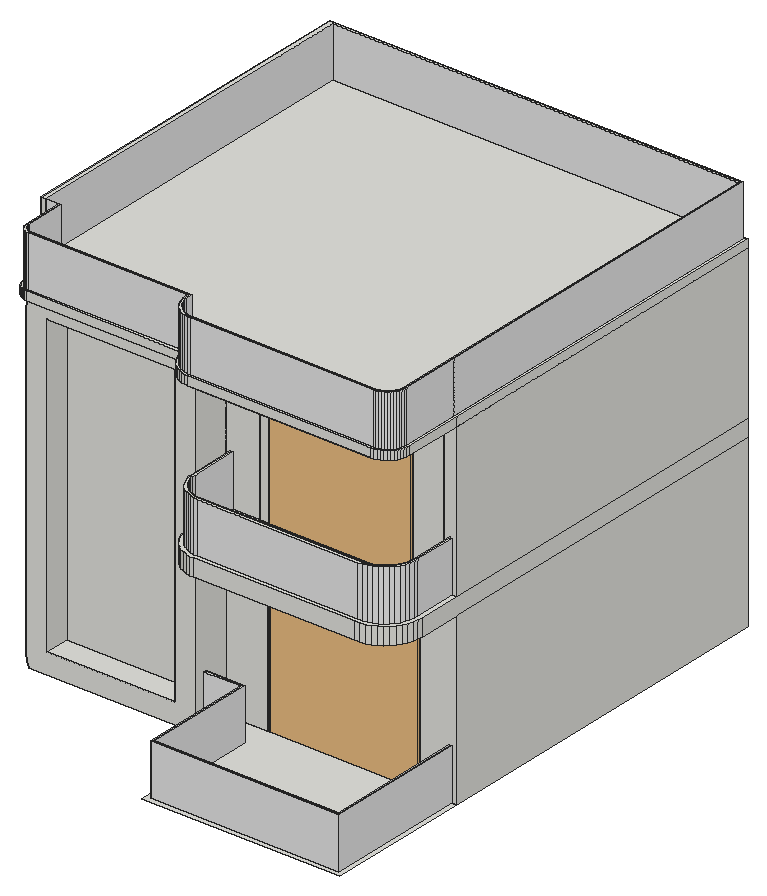
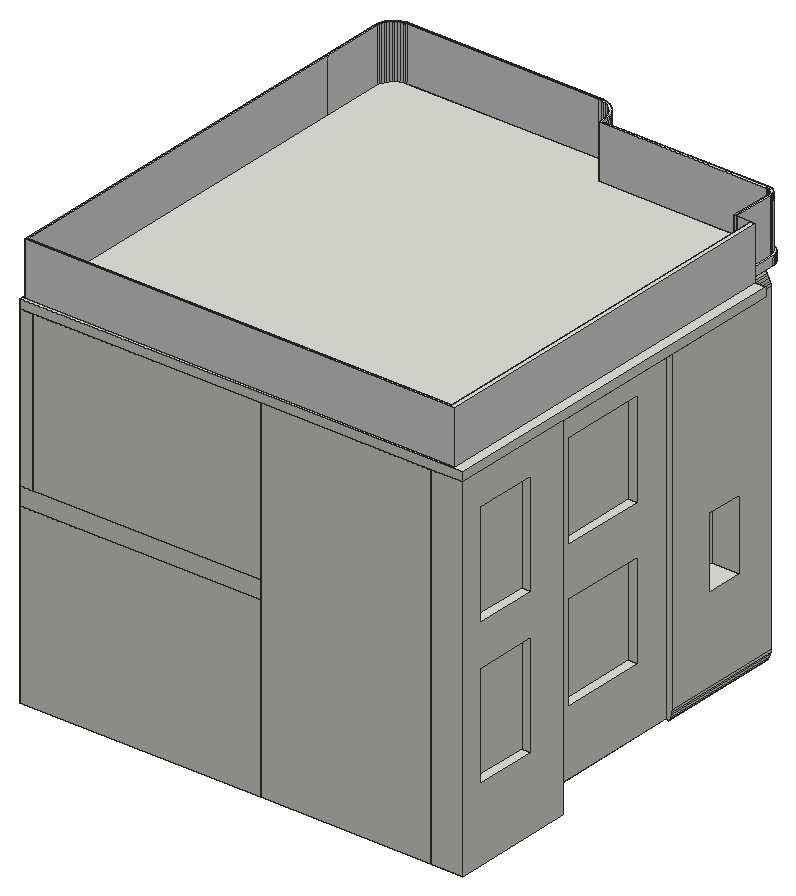
# SketchUp Ruby script. Lengths in inches.
U = 1.inch
M = Sketchup.active_model
def pt(a) = Geom::Point3d.new(a.map { |v| v * U })
def face(e, loops, mat)
  f = e.add_face(loops[0].map { |a| pt(a) })
  loops[1..].each { |l| e.add_face(l.map { |a| pt(a) }).erase! }
  f.material = f.back_material = mat if mat
  f
end
# faces: each face lists its corners as indices into pts; further lists are holes
def faces(e, pts, list, mat = nil) = list.each { |f| face(e, (f[0].is_a?(Array) ? f : [f]).map { |l| l.map { |i| pts[i] } }, mat) }
# xy, xz, yz: faces in a plane at the given z, y or x. An outline is a flat list of corners, or four numbers for a rectangle; further outlines are holes
def ring(l) = l.size == 4 ? [[l[0], l[1]], [l[2], l[1]], [l[2], l[3]], [l[0], l[3]]] : l.each_slice(2).to_a
def flat(e, list, mat, &to3) = list.each { |f| face(e, (f[0].is_a?(Array) ? f : [f]).map { |l| ring(l).map { |u, v| to3.(u, v) } }, mat) }
def xy(e, z, list, mat = nil) = flat(e, list, mat) { |x, y| [x, y, z] }
def xz(e, y, list, mat = nil) = flat(e, list, mat) { |x, z| [x, y, z] }
def yz(e, x, list, mat = nil) = flat(e, list, mat) { |y, z| [x, y, z] }
def lines(e, pts, list) = list.each { |a, b| e.add_line(pt(pts[a]), pt(pts[b])) }
# prism: a flat outline (further loops are holes) pulled along v
def prism(e, loops, v, mat = nil)
  f = face(e, loops, mat); d = Geom::Vector3d.new(v.map { |x| x * U })
  f.pushpull(f.normal.samedirection?(d) ? d.length : -d.length)
end
def box(e, o, s, mat = nil) = prism(e, [[o, [o[0] + s[0], o[1], o[2]], [o[0] + s[0], o[1] + s[1], o[2]], [o[0], o[1] + s[1], o[2]]]], [0, 0, s[2]], mat)
def at(x, y, z, deg = 0) = Geom::Transformation.translation(pt([x, y, z])) * Geom::Transformation.rotation(ORIGIN, Z_AXIS, deg.degrees)
def axes(o, x, y, z) = Geom::Transformation.new([*x, 0, *y, 0, *z, 0, *pt(o).to_a, 1])
def part(name) = M.definitions.add(name)
# library, detail: a bought-in or finely detailed component or shape, given as its bounding box
def library(name, o, s) = part(name).tap { |d| box(d.entities, o, s) }
def detail(e, o, s) = box(e.add_group.entities, o, s)
def put(e, d, t, mat = nil) = e.add_instance(d, t).tap { |i| i.material = mat if mat }
def group(e, t, mat = nil) = e.add_group.tap { |g| g.transformation = t; g.material = mat if mat }.entities
root = M.entities
M.materials.add("[Mirror 02]").color = [229, 229, 229]
c1 = library("Curtains 004",[-15.59,-2.26,0],[31.18,4.52,116.91])
c2 = library("Door 46-41",[-69.27,-3.71,0.02],[138.54,7.43,97.71])
xy(root,252,[[219.5625,0,360,0,360,102.93,356.5,102.93,356.5,3.5,223.0625,3.5,223.0625,83,196.57,83,196.57,79.5,219.5625,79.5],[223.0625,3.5,223.0625,83,196.57,83,196.57,84.76,224.82,84.76,224.82,5.26,354.74,5.26,354.74,102.93,356.5,102.93,356.5,3.5],[224.82,5.26,354.74,5.26,354.74,102.93,334.22,102.93,334.22,111.93,227.87,111.93,227.87,102.93,196.57,102.93,196.57,84.76,224.82,84.76],[196.57,102.93,196.57,360,360,360,360,102.93,334.22,102.93,334.22,111.93,351,111.93,351,351,205.57,351,205.57,111.93,227.87,111.93,227.87,102.93],[205.57,111.93,351,351],
  [81,159.75,196.57,275],[59.04,275,81,360],[81,275,196.57,360]])
xy(root,266.67,[[91.49,76.3125,181.9,93.625]])
xy(root,288,[[223.0625,3.5,356.5,3.5,356.5,102.93,354.74,102.93,354.74,5.26,224.82,5.26,224.82,84.76,196.57,84.76,196.57,83,223.0625,83]])
xy(root,296.33,[[81,184.12,87.625,242.93]])
xy(root,301.73,[[59.04,301.97,65.66,345.47]])
xy(root,316.9,[[76.8125,102.66,95.5625,128.53]])
xy(root,361.83,[[81,184.12,87.625,242.93]])
xy(root,365.21,[[76.8125,102.66,95.5625,128.53]])
xy(root,372,[[219.65,46.1875,216.64,46.38,213.67,46.97,210.82,47.94,208.11,49.28,205.6,50.96,203.33,52.95,201.34,55.22,199.66,57.73,198.33,60.43,197.36,63.29,196.77,66.25,196.57,69.27,196.57,102.93,227.87,102.93,227.87,111.93,205.57,111.93,205.57,351,351,351,351,111.93,334.22,111.93,334.22,102.93,360,102.93,360,72.79,359.77,69.32,359.09,65.9,357.98,62.61,356.4375,59.49,354.5,56.6,352.21,53.98,349.59,51.68,346.7,49.75,343.58,48.21,340.28,47.09,336.87,46.42,333.4,46.1875],[196.57,102.93,196.57,360,360,360,360,102.93,334.22,102.93,334.22,111.93,351,111.93,351,351,205.57,351,205.57,111.93,227.87,111.93,227.87,102.93]])
xy(root,372.12,[[59.04,301.97,65.66,345.47]])
xy(root,384,[[219.65,46.1875,333.4,46.1875,336.87,46.42,340.28,47.09,343.58,48.21,346.7,49.75,349.59,51.68,352.21,53.98,354.5,56.6,356.4375,59.49,357.98,62.61,359.09,65.9,359.77,69.32,360,72.79,360,102.8125,356.95,102.8125,356.95,72.79,356.74,69.72,356.14,66.69,355.15,63.78,353.79,61.02,352.08,58.45,350.05,56.14,347.73,54.11,345.17,52.4,342.41,51.03,339.49,50.04,336.47,49.44,333.4,49.24,219.65,49.24,217.03,49.41,214.47,49.92,211.98,50.77,209.64,51.92,207.46,53.38,205.49,55.11,203.76,57.08,202.31,59.25,201.15,61.6,200.31,64.08,199.79,66.65,199.625,69.27,199.625,102.8125,196.57,102.8125,196.57,69.27,196.77,66.25,197.36,63.29,198.33,60.43,199.66,57.73,201.34,55.22,203.33,52.95,205.6,50.96,208.11,49.28,210.82,47.94,213.67,46.97,216.64,46.38],[219.65,49.24,217.03,49.41,214.47,49.92,211.98,50.77,209.64,51.92,207.46,53.38,205.49,55.11,203.76,57.08,202.31,59.25,201.15,61.6,200.31,64.08,199.79,66.65,199.625,69.27,199.625,102.8125,201.5,102.8125,201.5,69.27,201.66,66.9,202.12,64.57,202.89,62.32,203.94,60.19,205.25,58.22,206.82,56.4375,208.6,54.87,210.58,53.55,212.7,52.5,214.95,51.74,217.28,51.28,219.65,51.12,333.4,51.12,336.23,51.31,339.01,51.86,341.69,52.77,344.23,54.02,346.59,55.6,348.72,57.47,350.59,59.6,352.16,61.96,353.42,64.5,354.33,67.18,354.88,69.96,355.07,72.79,355.07,102.8125,356.95,102.8125,356.95,72.79,356.74,69.72,356.14,66.69,355.15,63.78,353.79,61.02,352.08,58.45,350.05,56.14,347.73,54.11,345.17,52.4,342.41,51.03,339.49,50.04,336.47,49.44,333.4,49.24],[219.65,51.12,333.4,51.12,336.23,51.31,339.01,51.86,341.69,52.77,344.23,54.02,346.59,55.6,348.72,57.47,350.59,59.6,352.16,61.96,353.42,64.5,354.33,67.18,354.88,69.96,355.07,72.79,355.07,102.8125,329.25,102.8125,329.25,111.8125,227.25,111.8125,227.25,102.8125,201.5,102.8125,201.5,69.27,201.66,66.9,202.12,64.57,202.89,62.32,203.94,60.19,205.25,58.22,206.82,56.4375,208.6,54.87,210.58,53.55,212.7,52.5,214.95,51.74,217.28,51.28],[196.57,102.8125,227.25,111.8125],[329.25,102.8125,351,111.8125],
  [351,102.8125,360,360],[196.57,111.8125,351,351],[196.57,351,351,360]])
xy(root,394.46,[[81,184.12,87.625,242.93]])
xy(root,399.98,[[59.04,301.97,65.66,345.47]])
xy(root,420,[[219.65,49.24,333.4,49.24,336.47,49.44,339.49,50.04,342.41,51.03,345.17,52.4,347.73,54.11,350.05,56.14,352.08,58.45,353.79,61.02,355.15,63.78,356.14,66.69,356.74,69.72,356.95,72.79,356.95,102.8125,355.07,102.8125,355.07,72.79,354.88,69.96,354.33,67.18,353.42,64.5,352.16,61.96,350.59,59.6,348.72,57.47,346.59,55.6,344.23,54.02,341.69,52.77,339.01,51.86,336.23,51.31,333.4,51.12,219.65,51.12,217.28,51.28,214.95,51.74,212.7,52.5,210.58,53.55,208.6,54.87,206.82,56.4375,205.25,58.22,203.94,60.19,202.89,62.32,202.12,64.57,201.66,66.9,201.5,69.27,201.5,102.8125,199.625,102.8125,199.625,69.27,199.79,66.65,200.31,64.08,201.15,61.6,202.31,59.25,203.76,57.08,205.49,55.11,207.46,53.38,209.64,51.92,211.98,50.77,214.47,49.92,217.03,49.41]])
xy(root,459.96,[[81,184.12,87.625,242.93]])
xy(root,470.37,[[59.04,301.97,65.66,345.47]])
xy(root,474.75,[[227.25,102.8125,329.25,111.8125]])
xy(root,477.33,[[91.49,76.3125,181.9,93.625]])
xy(root,492,[[215.57,46.1875,213.09,46.35,210.65,46.83,208.3,47.63,206.07,48.73,204,50.11,202.13,51.75,200.5,53.62,199.12,55.6875,198.02,57.91,197.22,60.27,196.73,62.71,196.57,65.18,85.88,65.18,84.7,65.26,83.54,65.49,82.41,65.875,81.35,66.4,80.36,67.06,79.47,67.84,78.6875,68.73,78.03,69.72,77.5,70.78,77.12,71.91,76.89,73.07,76.8125,74.26,76.8125,102.8125,88.75,102.8125,88.75,76.3125,184.95,76.3125,184.95,102.8125,351,102.8125,351,47.44,350.77,47.33,348.91,46.7,347,46.32,345.04,46.1875],[351,47.44,351,102.8125,360,102.8125,360,61.14,359.87,59.19,359.49,57.27,358.86,55.42,358,53.67,356.91,52.04,355.62,50.57,354.15,49.28,352.52,48.19],[88.75,76.3125,184.95,102.8125],[88.75,76.3125,184.95,102.8125],[59.04,102.8125,88.75,111.8125],
  [88.75,102.8125,184.95,111.8125],[184.95,102.8125,196.57,111.8125],[196.57,102.8125,351,111.8125],[351,102.8125,360,360],[59.04,111.8125,88.75,159.75],
  [88.75,111.8125,184.95,159.75],[184.95,111.8125,184.95,159.75,196.57,159.75,196.57,351,351,351,351,111.8125],[59.04,159.75,81,275],[81,159.75,196.57,275],[59.04,275,81,351],
  [81,275,196.57,351],[59.04,351,81,360],[81,351,196.57,360],[196.57,351,351,360]])
xy(root,498,[[215.57,46.1875,345.04,46.1875,347,46.32,348.91,46.7,350.77,47.33,352.52,48.19,354.15,49.28,355.62,50.57,356.91,52.04,358,53.67,358.86,55.42,359.49,57.27,359.87,59.19,360,61.14,360,360,59.04,360,59.04,102.8125,66.02,102.8125,66.02,358.17,358.17,358.17,358.17,61.14,358.06,59.43,357.72,57.75,357.17,56.12,356.41,54.58,355.46,53.15,354.33,51.86,353.04,50.73,351.61,49.77,350.07,49.01,348.44,48.46,346.76,48.13,345.04,48.02,215.63,48.02,213.33,48.17,211.125,48.6,209,49.33,206.98,50.32,205.12,51.57,203.43,53.05,201.95,54.74,200.7,56.6,199.71,58.62,198.99,60.74,198.55,62.94,198.28,67.01,85.88,67.01,84.9375,67.07,84.01,67.26,83.11,67.5625,82.26,67.98,81.47,68.51,80.76,69.13,80.14,69.85,79.61,70.63,79.19,71.48,78.89,72.38,78.7,73.3125,78.64,74.26,78.64,102.8125,76.8125,102.8125,76.8125,74.26,76.89,73.07,77.12,71.91,77.5,70.78,78.03,69.72,78.6875,68.73,79.47,67.84,80.36,67.06,81.35,66.4,82.41,65.875,83.54,65.49,84.7,65.26,85.88,65.18,196.57,65.18,196.73,62.71,197.22,60.27,198.02,57.91,199.12,55.6875,200.5,53.62,202.13,51.75,204,50.11,206.07,48.73,208.3,47.63,210.65,46.83,213.09,46.35],[215.63,48.02,213.33,48.17,211.125,48.6,209,49.33,206.98,50.32,205.12,51.57,203.43,53.05,201.95,54.74,200.7,56.6,199.71,58.62,198.99,60.74,198.55,62.94,198.28,67.01,85.88,67.01,84.9375,67.07,84.01,67.26,83.11,67.5625,82.26,67.98,81.47,68.51,80.76,69.13,80.14,69.85,79.61,70.63,79.19,71.48,78.89,72.38,78.7,73.3125,78.64,74.26,78.64,102.8125,80.33,102.8125,80.33,74.26,80.38,73.53,80.52,72.82,80.75,72.13,81.08,71.48,81.48,70.875,81.96,70.33,82.5,69.85,83.11,69.45,83.76,69.125,84.45,68.89,85.16,68.75,85.88,68.7,199.87,68.7,200.23,63.17,200.625,61.18,201.27,59.26,202.17,57.45,203.29,55.77,204.63,54.25,206.15,52.91,207.83,51.79,209.65,50.89,211.5625,50.24,213.55,49.85,215.68,49.71,345.04,49.71,346.54,49.8,348,50.1,349.42,50.58,350.76,51.24,352.01,52.07,353.13,53.06,354.12,54.18,354.95,55.43,355.61,56.77,356.09,58.18,356.38,59.65,356.48,61.14,356.48,356.48,69.33,356.48,69.33,102.8125,66.02,102.8125,66.02,358.17,358.17,358.17,358.17,61.14,358.06,59.43,357.72,57.75,357.17,56.12,356.41,54.58,355.46,53.15,354.33,51.86,353.04,50.73,351.61,49.77,350.07,49.01,348.44,48.46,346.76,48.13,345.04,48.02],[215.68,49.71,345.04,49.71,346.54,49.8,348,50.1,349.42,50.58,350.76,51.24,352.01,52.07,353.13,53.06,354.12,54.18,354.95,55.43,355.61,56.77,356.09,58.18,356.38,59.65,356.48,61.14,356.48,356.48,69.33,356.48,69.33,102.8125,80.33,102.8125,80.33,74.26,80.38,73.53,80.52,72.82,80.75,72.13,81.08,71.48,81.48,70.875,81.96,70.33,82.5,69.85,83.11,69.45,83.76,69.125,84.45,68.89,85.16,68.75,85.88,68.7,199.87,68.7,200.23,63.17,200.625,61.18,201.27,59.26,202.17,57.45,203.29,55.77,204.63,54.25,206.15,52.91,207.83,51.79,209.65,50.89,211.5625,50.24,213.55,49.85]])
xy(root,534,[[215.63,48.02,345.04,48.02,346.76,48.13,348.44,48.46,350.07,49.01,351.61,49.77,353.04,50.73,354.33,51.86,355.46,53.15,356.41,54.58,357.17,56.12,357.72,57.75,358.06,59.43,358.17,61.14,358.17,358.17,66.02,358.17,66.02,102.8125,69.33,102.8125,69.33,356.48,356.48,356.48,356.48,61.14,356.38,59.65,356.09,58.18,355.61,56.77,354.95,55.43,354.12,54.18,353.13,53.06,352.01,52.07,350.76,51.24,349.42,50.58,348,50.1,346.54,49.8,345.04,49.71,215.68,49.71,213.55,49.85,211.5625,50.24,209.65,50.89,207.83,51.79,206.15,52.91,204.63,54.25,203.29,55.77,202.17,57.45,201.27,59.26,200.625,61.18,200.23,63.17,199.87,68.7,85.88,68.7,85.16,68.75,84.45,68.89,83.76,69.125,83.11,69.45,82.5,69.85,81.96,70.33,81.48,70.875,81.08,71.48,80.75,72.13,80.52,72.82,80.38,73.53,80.33,74.26,80.33,102.8125,78.64,102.8125,78.64,74.26,78.7,73.3125,78.89,72.38,79.19,71.48,79.61,70.63,80.14,69.85,80.76,69.13,81.47,68.51,82.26,67.98,83.11,67.5625,84.01,67.26,84.9375,67.07,85.88,67.01,198.28,67.01,198.55,62.94,198.99,60.74,199.71,58.62,200.7,56.6,201.95,54.74,203.43,53.05,205.12,51.57,206.98,50.32,209,49.33,211.125,48.6,213.33,48.17]])
xz(root,3.5,[[223.0625,252,356.5,288]],"[Mirror 02]")
xz(root,5.26,[[224.82,252,354.74,288]],"[Mirror 02]")
xz(root,46.1875,[[219.65,372,333.4,384],[215.57,492,345.04,498]])
xz(root,48.02,[[215.63,498,345.04,534]],"[Mirror 02]")
xz(root,49.24,[[219.65,384,333.4,420]],"[Mirror 02]")
xz(root,49.71,[[215.68,498,345.04,534]],"[Mirror 02]")
xz(root,51.12,[[219.65,384,333.4,420]],"[Mirror 02]")
xz(root,65.18,[[85.88,492,196.57,498]])
xz(root,67.01,[[85.88,498,198.28,534]],"[Mirror 02]")
xz(root,68.7,[[85.88,498,199.87,534]],"[Mirror 02]")
xz(root,76.3125,[[[78.98,252,194.59,252,195.01,252.63,195.69,254.01,196.22,255.46,196.57,256.96,196.57,480.38,196.47,481.9,196.17,483.39,195.69,484.83,195.01,486.1875,194.17,487.45,193.17,488.6,192.02,489.6,190.76,490.44,189.4,491.12,187.96,491.6,186.47,491.9,184.95,492,88.75,492,87.19,491.9,85.66,491.59,84.18,491.09,82.78,490.4,81.48,489.53,80.31,488.5,79.28,487.33,78.41,486.03,77.72,484.63,77.22,483.15,76.91,481.62,76.8125,480.06,76.8125,259.1875,76.93,257.47,77.26,255.77,77.82,254.14,78.58,252.59],[91.49,266.67,181.9,477.33]]])
xz(root,83,[[196.57,252,223.0625,288]],"[Mirror 02]")
xz(root,84.76,[[196.57,252,224.82,288]],"[Mirror 02]")
xz(root,93.625,[[91.49,266.67,181.9,477.33]])
xz(root,102.66,[[76.8125,316.9,95.5625,365.21]])
xz(root,102.8125,[[196.57,384,199.625,384,199.625,420,201.5,420,201.5,384,227.25,384,227.25,474.75,329.25,474.75,329.25,384,351,384,351,492,196.57,492],[199.625,384,201.5,420],[351,384,355.07,384,355.07,420,356.95,420,356.95,384,360,384,360,492,351,492],[355.07,384,356.95,420],[59.04,492,76.8125,498],
  [66.02,498,69.33,534]])
xz(root,102.8125,[[69.33,498,78.64,534],[78.64,498,80.33,534]],"[Mirror 02]")
xz(root,102.93,[[196.57,252,227.87,372],[334.22,252,354.74,252,354.74,288,356.5,288,356.5,252,360,252,360,372,334.22,372],[354.74,252,356.5,288]])
xz(root,111.8125,[[196.57,384,196.57,492,351,492,351,384,329.25,384,329.25,474.75,227.25,474.75,227.25,384]])
xz(root,111.93,[[205.57,252,227.87,372],[334.22,252,351,372]])
xz(root,128.53,[[76.8125,316.9,95.5625,365.21]])
xz(root,159.75,[[78.98,252,78.58,252.59,77.82,254.14,77.26,255.77,76.93,257.47,76.8125,259.1875,76.8125,480.06,76.91,481.62,77.22,483.15,77.72,484.63,78.41,486.03,79.28,487.33,80.31,488.5,81,489.11,81,252],[81,252,81,489.11,81.48,489.53,82.78,490.4,84.18,491.09,85.66,491.59,87.19,491.9,88.75,492,184.95,492,186.47,491.9,187.96,491.6,189.4,491.12,190.76,490.44,192.02,489.6,193.17,488.6,194.17,487.45,195.01,486.1875,195.69,484.83,196.17,483.39,196.47,481.9,196.57,480.38,196.57,252],[196.57,480.38,196.57,492,184.95,492,186.47,491.9,187.96,491.6,189.4,491.12,190.76,490.44,192.02,489.6,193.17,488.6,194.17,487.45,195.01,486.1875,195.69,484.83,196.17,483.39,196.47,481.9],[81,489.11,81.48,489.53,82.78,490.4,84.18,491.09,85.66,491.59,87.19,491.9,88.75,492,81,492]])
xz(root,184.12,[[81,296.33,87.625,361.83],[81,394.46,87.625,459.96]])
xz(root,242.93,[[81,296.33,87.625,361.83],[81,394.46,87.625,459.96]])
xz(root,275,[[59.04,252,81,492],[81,252,196.57,492]])
xz(root,301.97,[[59.04,301.73,65.66,372.12],[59.04,399.98,65.66,470.37]])
xz(root,345.47,[[59.04,301.73,65.66,372.12],[59.04,399.98,65.66,470.37]])
xz(root,351,[[205.57,252,351,372],[196.57,384,351,492]])
xz(root,356.48,[[69.33,498,356.48,534]],"[Mirror 02]")
xz(root,358.17,[[66.02,498,358.17,534]],"[Mirror 02]")
xz(root,360,[[59.04,252,81,492],[81,252,196.57,492],[196.57,252,360,372],[196.57,372,360,384],[196.57,384,351,492],
  [351,384,360,492],[59.04,492,360,498]])
yz(root,59.04,[[[275,252,360,492],[301.97,399.98,345.47,470.37],[301.97,301.73,345.47,372.12]],[102.8125,492,360,498]])
yz(root,65.66,[[301.97,301.73,345.47,372.12],[301.97,399.98,345.47,470.37]])
yz(root,66.02,[[102.8125,498,358.17,534]],"[Mirror 02]")
yz(root,69.33,[[102.8125,498,356.48,534]],"[Mirror 02]")
yz(root,76.8125,[[[76.3125,259.1875,159.75,480.06],[102.66,316.9,128.53,365.21]],[74.26,492,102.8125,498]])
yz(root,78.64,[[74.26,498,102.8125,534]],"[Mirror 02]")
yz(root,80.33,[[74.26,498,102.8125,534]],"[Mirror 02]")
yz(root,81,[[[159.75,252,248.24,492],[184.12,394.46,242.93,459.96],[184.12,296.33,242.93,361.83]],[248.24,252,275,492],[275,252,360,492]])
yz(root,87.625,[[184.12,296.33,242.93,361.83],[184.12,394.46,242.93,459.96]])
yz(root,91.49,[[76.3125,266.67,93.625,477.33]])
yz(root,95.5625,[[102.66,316.9,128.53,365.21]])
yz(root,181.9,[[76.3125,266.67,93.625,477.33]])
yz(root,196.57,[[79.5,252,83,252,83,288,84.76,288,84.76,252,102.93,252,102.93,372,76.3125,372,76.3125,256.96,79.5,256.96],[83,252,84.76,288],[102.93,252,159.75,372],[159.75,252,275,372],[275,252,360,372],
  [69.27,372,76.3125,384],[76.3125,372,159.75,384],[159.75,372,275,384],[275,372,360,384],[76.3125,384,102.8125,480.38],
  [102.8125,384,111.8125,480.38],[111.8125,384,159.75,480.38],[159.75,384,275,492],[275,384,351,492],[351,384,360,492],
  [102.8125,480.38,111.8125,492]])
yz(root,199.625,[[69.27,384,76.3125,420],[76.3125,384,102.8125,420]],"[Mirror 02]")
yz(root,201.5,[[69.27,384,102.8125,420]],"[Mirror 02]")
yz(root,205.57,[[111.93,252,159.75,372],[159.75,252,351,372]])
yz(root,223.0625,[[3.5,252,83,288]],"[Mirror 02]")
yz(root,224.82,[[5.26,252,84.76,288]],"[Mirror 02]")
yz(root,227.25,[[102.8125,384,111.8125,474.75]])
yz(root,227.87,[[102.93,252,111.93,372]])
yz(root,329.25,[[102.8125,384,111.8125,474.75]])
yz(root,334.22,[[102.93,252,111.93,372]])
yz(root,351,[[111.93,252,351,372],[102.8125,384,111.8125,492],[111.8125,384,351,492],[351,384,360,492]])
yz(root,354.74,[[5.26,252,102.93,288]],"[Mirror 02]")
yz(root,355.07,[[72.79,384,102.8125,420]],"[Mirror 02]")
yz(root,356.48,[[61.14,498,102.8125,534],[102.8125,498,356.48,534]],"[Mirror 02]")
yz(root,356.5,[[3.5,252,102.93,288]],"[Mirror 02]")
yz(root,356.95,[[72.79,384,102.8125,420]],"[Mirror 02]")
yz(root,358.17,[[61.14,498,102.8125,534],[102.8125,498,358.17,534]],"[Mirror 02]")
yz(root,360,[[102.93,252,360,372],[72.79,372,360,384],[102.8125,384,360,492],[61.14,492,102.8125,498],[102.8125,492,360,498]])
p = [[78.98,76.3125,252],[78.58,76.3125,252.59],[78.58,159.75,252.59],[78.98,159.75,252],[195.01,76.3125,252.63],[194.59,76.3125,252],
  [194.59,79.5,252],[195.01,79.5,252.63],[77.82,76.3125,254.14],[77.82,159.75,254.14],[195.69,76.3125,254.01],[195.69,79.5,254.01],
  [196.22,76.3125,255.46],[196.22,79.5,255.46],[77.26,76.3125,255.77],[77.26,159.75,255.77],[196.57,76.3125,256.96],[196.57,79.5,256.96],
  [76.93,76.3125,257.47],[76.93,159.75,257.47],[76.8125,76.3125,259.1875],[76.8125,159.75,259.1875],[219.65,46.1875,384],[216.64,46.38,384],
  [216.64,46.38,372],[219.65,46.1875,372],[336.87,46.42,384],[333.4,46.1875,384],[333.4,46.1875,372],[336.87,46.42,372],
  [213.67,46.97,384],[213.67,46.97,372],[340.28,47.09,384],[340.28,47.09,372],[210.82,47.94,384],[210.82,47.94,372],
  [343.58,48.21,384],[343.58,48.21,372],[208.11,49.28,384],[208.11,49.28,372],[346.7,49.75,384],[346.7,49.75,372],
  [205.6,50.96,384],[205.6,50.96,372],[349.59,51.68,384],[349.59,51.68,372],[203.33,52.95,384],[203.33,52.95,372],
  [352.21,53.98,384],[352.21,53.98,372],[201.34,55.22,384],[201.34,55.22,372],[354.5,56.6,384],[354.5,56.6,372],
  [199.66,57.73,384],[199.66,57.73,372],[356.4375,59.49,384],[356.4375,59.49,372],[198.33,60.43,384],[198.33,60.43,372],
  [357.98,62.61,384],[357.98,62.61,372],[197.36,63.29,384],[197.36,63.29,372],[359.09,65.9,384],[359.09,65.9,372],
  [196.77,66.25,384],[196.77,66.25,372],[359.77,69.32,384],[359.77,69.32,372],[196.57,69.27,384],[196.57,69.27,372],
  [360,72.79,384],[360,72.79,372],[217.03,49.41,384],[219.65,49.24,384],[219.65,49.24,420],[217.03,49.41,420],
  [333.4,49.24,384],[336.47,49.44,384],[336.47,49.44,420],[333.4,49.24,420],[214.47,49.92,384],[214.47,49.92,420],
  [339.49,50.04,384],[339.49,50.04,420],[211.98,50.77,384],[211.98,50.77,420],[342.41,51.03,384],[342.41,51.03,420],
  [209.64,51.92,384],[209.64,51.92,420],[345.17,52.4,384],[345.17,52.4,420],[219.65,51.12,384],[217.28,51.28,384],
  [217.28,51.28,420],[219.65,51.12,420],[336.23,51.31,384],[333.4,51.12,384],[333.4,51.12,420],[336.23,51.31,420],
  [214.95,51.74,384],[214.95,51.74,420],[339.01,51.86,384],[339.01,51.86,420],[212.7,52.5,384],[212.7,52.5,420],
  [207.46,53.38,384],[207.46,53.38,420],[341.69,52.77,384],[341.69,52.77,420],[347.73,54.11,384],[347.73,54.11,420],
  [210.58,53.55,384],[210.58,53.55,420],[344.23,54.02,384],[344.23,54.02,420],[205.49,55.11,384],[205.49,55.11,420],
  [208.6,54.87,384],[208.6,54.87,420],[346.59,55.6,384],[346.59,55.6,420],[350.05,56.14,384],[350.05,56.14,420],
  [206.82,56.4375,384],[206.82,56.4375,420],[203.76,57.08,384],[203.76,57.08,420],[348.72,57.47,384],[348.72,57.47,420],
  [352.08,58.45,384],[352.08,58.45,420],[205.25,58.22,384],[205.25,58.22,420],[202.31,59.25,384],[202.31,59.25,420],
  [350.59,59.6,384],[350.59,59.6,420],[203.94,60.19,384],[203.94,60.19,420],[353.79,61.02,384],[353.79,61.02,420],
  [201.15,61.6,384],[201.15,61.6,420],[352.16,61.96,384],[352.16,61.96,420],[202.89,62.32,384],[202.89,62.32,420],
  [355.15,63.78,384],[355.15,63.78,420],[200.31,64.08,384],[200.31,64.08,420],[353.42,64.5,384],[353.42,64.5,420],
  [202.12,64.57,384],[202.12,64.57,420],[356.14,66.69,384],[356.14,66.69,420],[199.79,66.65,384],[199.79,66.65,420],
  [354.33,67.18,384],[354.33,67.18,420],[201.66,66.9,384],[201.66,66.9,420],[199.625,69.27,384],[199.625,69.27,420],
  [356.74,69.72,384],[356.74,69.72,420],[201.5,69.27,384],[201.5,69.27,420],[354.88,69.96,384],[354.88,69.96,420],
  [356.95,72.79,384],[356.95,72.79,420],[355.07,72.79,384],[355.07,72.79,420],[76.8125,76.3125,480.06],[76.91,76.3125,481.62],
  [76.91,159.75,481.62],[76.8125,159.75,480.06],[196.47,76.3125,481.9],[196.57,76.3125,480.38],[196.57,102.8125,480.38],[196.57,111.8125,480.38],
  [196.57,159.75,480.38],[196.47,159.75,481.9],[77.22,76.3125,483.15],[77.22,159.75,483.15],[196.17,76.3125,483.39],[196.17,159.75,483.39],
  [77.72,76.3125,484.63],[77.72,159.75,484.63],[195.69,76.3125,484.83],[195.69,159.75,484.83],[78.41,76.3125,486.03],[78.41,159.75,486.03],
  [195.01,76.3125,486.1875],[195.01,159.75,486.1875],[79.28,76.3125,487.33],[79.28,159.75,487.33],[194.17,76.3125,487.45],[194.17,159.75,487.45],
  [80.31,76.3125,488.5],[80.31,159.75,488.5],[193.17,76.3125,488.6],[193.17,159.75,488.6],[81.48,76.3125,489.53],[81.48,159.75,489.53],
  [81,159.75,489.11],[192.02,76.3125,489.6],[192.02,159.75,489.6],[82.78,76.3125,490.4],[82.78,159.75,490.4],[190.76,76.3125,490.44],
  [190.76,159.75,490.44],[84.18,76.3125,491.09],[84.18,159.75,491.09],[189.4,76.3125,491.12],[189.4,159.75,491.12],[85.66,76.3125,491.59],
  [85.66,159.75,491.59],[187.96,76.3125,491.6],[187.96,159.75,491.6],[87.19,76.3125,491.9],[87.19,159.75,491.9],[186.47,76.3125,491.9],
  [186.47,159.75,491.9],[88.75,76.3125,492],[88.75,102.8125,492],[88.75,111.8125,492],[88.75,159.75,492],[184.95,76.3125,492],
  [184.95,159.75,492],[184.95,111.8125,492],[184.95,102.8125,492],[215.57,46.1875,498],[213.09,46.35,498],[213.09,46.35,492],
  [215.57,46.1875,492],[347,46.32,498],[345.04,46.1875,498],[345.04,46.1875,492],[347,46.32,492],[348.91,46.7,498],
  [348.91,46.7,492],[210.65,46.83,498],[210.65,46.83,492],[350.77,47.33,498],[350.77,47.33,492],[208.3,47.63,498],
  [208.3,47.63,492],[352.52,48.19,498],[351,47.44,492],[352.52,48.19,492],[206.07,48.73,498],[206.07,48.73,492],
  [354.15,49.28,498],[354.15,49.28,492],[204,50.11,498],[204,50.11,492],[355.62,50.57,498],[355.62,50.57,492],
  [202.13,51.75,498],[202.13,51.75,492],[356.91,52.04,498],[356.91,52.04,492],[200.5,53.62,498],[200.5,53.62,492],
  [358,53.67,498],[358,53.67,492],[199.12,55.6875,498],[199.12,55.6875,492],[358.86,55.42,498],[358.86,55.42,492],
  [359.49,57.27,498],[359.49,57.27,492],[198.02,57.91,498],[198.02,57.91,492],[359.87,59.19,498],[359.87,59.19,492],
  [197.22,60.27,498],[197.22,60.27,492],[360,61.14,498],[360,61.14,492],[196.73,62.71,498],[196.73,62.71,492],
  [196.57,65.18,498],[196.57,65.18,492],[85.88,65.18,498],[84.7,65.26,498],[84.7,65.26,492],[85.88,65.18,492],
  [83.54,65.49,498],[83.54,65.49,492],[82.41,65.875,498],[82.41,65.875,492],[81.35,66.4,498],[81.35,66.4,492],
  [80.36,67.06,498],[80.36,67.06,492],[79.47,67.84,498],[79.47,67.84,492],[78.6875,68.73,498],[78.6875,68.73,492],
  [78.03,69.72,498],[78.03,69.72,492],[77.5,70.78,498],[77.5,70.78,492],[77.12,71.91,498],[77.12,71.91,492],
  [76.89,73.07,498],[76.89,73.07,492],[76.8125,74.26,498],[76.8125,74.26,492],[213.33,48.17,498],[215.63,48.02,498],
  [215.63,48.02,534],[213.33,48.17,534],[345.04,48.02,498],[346.76,48.13,498],[346.76,48.13,534],[345.04,48.02,534],
  [348.44,48.46,498],[348.44,48.46,534],[211.125,48.6,498],[211.125,48.6,534],[350.07,49.01,498],[350.07,49.01,534],
  [209,49.33,498],[209,49.33,534],[351.61,49.77,498],[351.61,49.77,534],[206.98,50.32,498],[206.98,50.32,534],
  [215.68,49.71,498],[213.55,49.85,498],[213.55,49.85,534],[215.68,49.71,534],[346.54,49.8,498],[345.04,49.71,498],
  [345.04,49.71,534],[346.54,49.8,534],[211.5625,50.24,498],[211.5625,50.24,534],[348,50.1,498],[348,50.1,534],
  [353.04,50.73,498],[353.04,50.73,534],[349.42,50.58,498],[349.42,50.58,534],[209.65,50.89,498],[209.65,50.89,534],
  [205.12,51.57,498],[205.12,51.57,534],[350.76,51.24,498],[350.76,51.24,534],[354.33,51.86,498],[354.33,51.86,534],
  [207.83,51.79,498],[207.83,51.79,534],[352.01,52.07,498],[352.01,52.07,534],[203.43,53.05,498],[203.43,53.05,534],
  [206.15,52.91,498],[206.15,52.91,534],[355.46,53.15,498],[355.46,53.15,534],[353.13,53.06,498],[353.13,53.06,534],
  [204.63,54.25,498],[204.63,54.25,534],[201.95,54.74,498],[201.95,54.74,534],[354.12,54.18,498],[354.12,54.18,534],
  [356.41,54.58,498],[356.41,54.58,534],[203.29,55.77,498],[203.29,55.77,534],[354.95,55.43,498],[354.95,55.43,534],
  [357.17,56.12,498],[357.17,56.12,534],[200.7,56.6,498],[200.7,56.6,534],[355.61,56.77,498],[355.61,56.77,534],
  [202.17,57.45,498],[202.17,57.45,534],[357.72,57.75,498],[357.72,57.75,534],[199.71,58.62,498],[199.71,58.62,534],
  [356.09,58.18,498],[356.09,58.18,534],[201.27,59.26,498],[201.27,59.26,534],[358.06,59.43,498],[358.06,59.43,534],
  [356.38,59.65,498],[356.38,59.65,534],[198.99,60.74,498],[198.99,60.74,534],[200.625,61.18,498],[200.625,61.18,534],
  [358.17,61.14,498],[358.17,61.14,534],[356.48,61.14,498],[356.48,61.14,534],[198.55,62.94,498],[198.55,62.94,534],
  [200.23,63.17,498],[200.23,63.17,534],[198.28,67.01,498],[198.28,67.01,534],[199.87,68.7,498],[199.87,68.7,534],
  [84.9375,67.07,498],[85.88,67.01,498],[85.88,67.01,534],[84.9375,67.07,534],[84.01,67.26,498],[84.01,67.26,534],
  [83.11,67.5625,498],[83.11,67.5625,534],[82.26,67.98,498],[82.26,67.98,534],[81.47,68.51,498],[81.47,68.51,534],
  [80.76,69.13,498],[80.76,69.13,534],[85.88,68.7,498],[85.16,68.75,498],[85.16,68.75,534],[85.88,68.7,534],
  [84.45,68.89,498],[84.45,68.89,534],[83.76,69.125,498],[83.76,69.125,534],[80.14,69.85,498],[80.14,69.85,534],
  [83.11,69.45,498],[83.11,69.45,534],[82.5,69.85,498],[82.5,69.85,534],[79.61,70.63,498],[79.61,70.63,534],
  [81.96,70.33,498],[81.96,70.33,534],[81.48,70.875,498],[81.48,70.875,534],[79.19,71.48,498],[79.19,71.48,534],
  [81.08,71.48,498],[81.08,71.48,534],[78.89,72.38,498],[78.89,72.38,534],[80.75,72.13,498],[80.75,72.13,534],
  [80.52,72.82,498],[80.52,72.82,534],[78.7,73.3125,498],[78.7,73.3125,534],[80.38,73.53,498],[80.38,73.53,534],
  [78.64,74.26,498],[78.64,74.26,534],[80.33,74.26,498],[80.33,74.26,534],[328.96,106.67,252],[233.13,106.67,252],
  [330.72,108.43,252],[231.37,108.43,252],[324.3125,106.88,384],[232.18,106.88,384],[326.2,108.76,384],[230.3,108.76,384]]
faces(root,p,[[0,1,2,3],[4,5,6,7],[1,8,9,2],[10,4,7,11],[12,10,11,13],[8,14,15,9],[16,12,13,17],[14,18,19,15],
  [18,20,21,19],[22,23,24,25],[26,27,28,29],[23,30,31,24],[32,26,29,33],[30,34,35,31],[36,32,33,37],[34,38,39,35],
  [40,36,37,41],[38,42,43,39],[44,40,41,45],[42,46,47,43],[48,44,45,49],[46,50,51,47],[52,48,49,53],[50,54,55,51],
  [56,52,53,57],[54,58,59,55],[60,56,57,61],[58,62,63,59],[64,60,61,65],[62,66,67,63],[68,64,65,69],[66,70,71,67],
  [72,68,69,73],[178,179,180,181],[182,183,184,185,186,187],[179,188,189,180],[190,182,187,191],[188,192,193,189],[194,190,191,195],[192,196,197,193],
  [198,194,195,199],[196,200,201,197],[202,198,199,203],[200,204,205,201],[206,202,203,207],[204,208,209,210,205],[211,206,207,212],[208,213,214,209],
  [215,211,212,216],[213,217,218,214],[219,215,216,220],[217,221,222,218],[223,219,220,224],[221,225,226,222],[227,223,224,228],[225,229,230,231,232,226],
  [233,227,228,234,235,236],[237,238,239,240],[241,242,243,244],[245,241,244,246],[238,247,248,239],[249,245,246,250],[247,251,252,248],[253,249,250,254,255],
  [251,256,257,252],[258,253,255,259],[256,260,261,257],[262,258,259,263],[260,264,265,261],[266,262,263,267],[264,268,269,265],[270,266,267,271],
  [268,272,273,269],[274,270,271,275],[276,274,275,277],[272,278,279,273],[280,276,277,281],[278,282,283,279],[284,280,281,285],[282,286,287,283],
  [286,288,289,287],[290,291,292,293],[291,294,295,292],[294,296,297,295],[296,298,299,297],[298,300,301,299],[300,302,303,301],[302,304,305,303],
  [304,306,307,305],[306,308,309,307],[308,310,311,309],[310,312,313,311],[312,314,315,313]])
faces(root,p,[[74,75,76,77],[78,79,80,81],[82,74,77,83],[79,84,85,80],[86,82,83,87],[84,88,89,85],[90,86,87,91],[88,92,93,89],
  [94,95,96,97],[98,99,100,101],[95,102,103,96],[104,98,101,105],[102,106,107,103],[108,90,91,109],[110,104,105,111],[92,112,113,93],
  [106,114,115,107],[116,110,111,117],[118,108,109,119],[114,120,121,115],[122,116,117,123],[112,124,125,113],[120,126,127,121],[128,118,119,129],
  [130,122,123,131],[124,132,133,125],[126,134,135,127],[136,128,129,137],[138,130,131,139],[134,140,141,135],[132,142,143,133],[144,136,137,145],
  [146,138,139,147],[140,148,149,141],[142,150,151,143],[152,144,145,153],[154,146,147,155],[148,156,157,149],[150,158,159,151],[160,152,153,161],
  [162,154,155,163],[156,164,165,157],[166,160,161,167],[158,168,169,159],[164,170,171,165],[172,162,163,173],[168,174,175,169],[176,172,173,177],
  [316,317,318,319],[320,321,322,323],[321,324,325,322],[326,316,319,327],[324,328,329,325],[330,326,327,331],[328,332,333,329],[334,330,331,335],
  [336,337,338,339],[340,341,342,343],[337,344,345,338],[346,340,343,347],[332,348,349,333],[350,346,347,351],[344,352,353,345],[354,334,335,355],
  [356,350,351,357],[348,358,359,349],[352,360,361,353],[362,356,357,363],[364,354,355,365],[360,366,367,361],[358,368,369,359],[370,362,363,371],
  [366,372,373,367],[374,364,365,375],[376,370,371,377],[368,378,379,369],[372,380,381,373],[382,376,377,383],[378,384,385,379],[386,374,375,387],
  [388,382,383,389],[380,390,391,381],[384,392,393,385],[394,386,387,395],[396,388,389,397],[390,398,399,391],[392,400,401,393],[402,396,397,403],
  [404,394,395,405],[398,406,407,399],[400,408,409,401],[410,402,403,411],[412,404,405,413],[406,414,415,407],[416,412,413,417],[414,418,419,415],
  [420,421,422,423],[424,420,423,425],[426,424,425,427],[428,426,427,429],[430,428,429,431],[432,430,431,433],[434,435,436,437],[435,438,439,436],
  [438,440,441,439],[442,432,433,443],[440,444,445,441],[444,446,447,445],[448,442,443,449],[446,450,451,447],[450,452,453,451],[454,448,449,455],
  [452,456,457,453],[458,454,455,459],[456,460,461,457],[460,462,463,461],[464,458,459,465],[462,466,467,463],[468,464,465,469],[466,470,471,467]],"[Mirror 02]")
lines(root,p,[[472,473],[474,475],[476,477],[478,479]])
put(root,c1,at(320.3125,115.3125,252))
put(root,c1,at(241.34,115.5,252))
put(root,c2,axes([279.4375,106.68,251.99],[0.77,0,0],[0,1,0],[0,0,1.22814]))
put(root,c2,axes([274.47,106.5625,384],[0.77,0,0],[0,1,0],[0,0,0.92847]))
